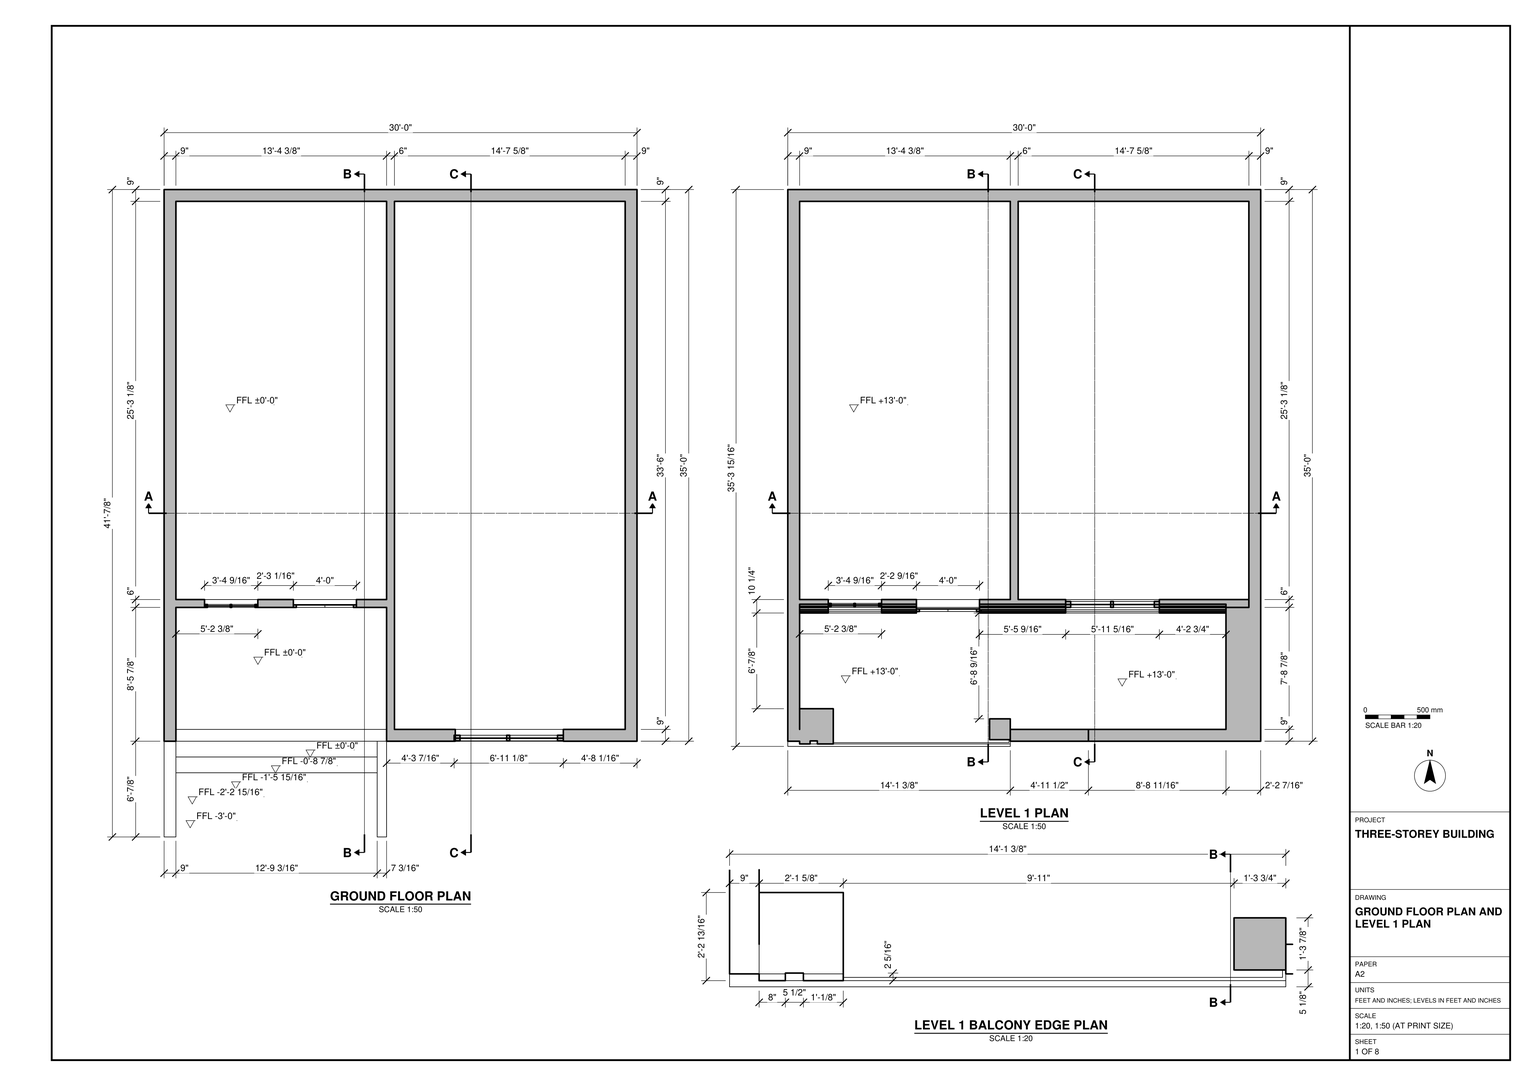
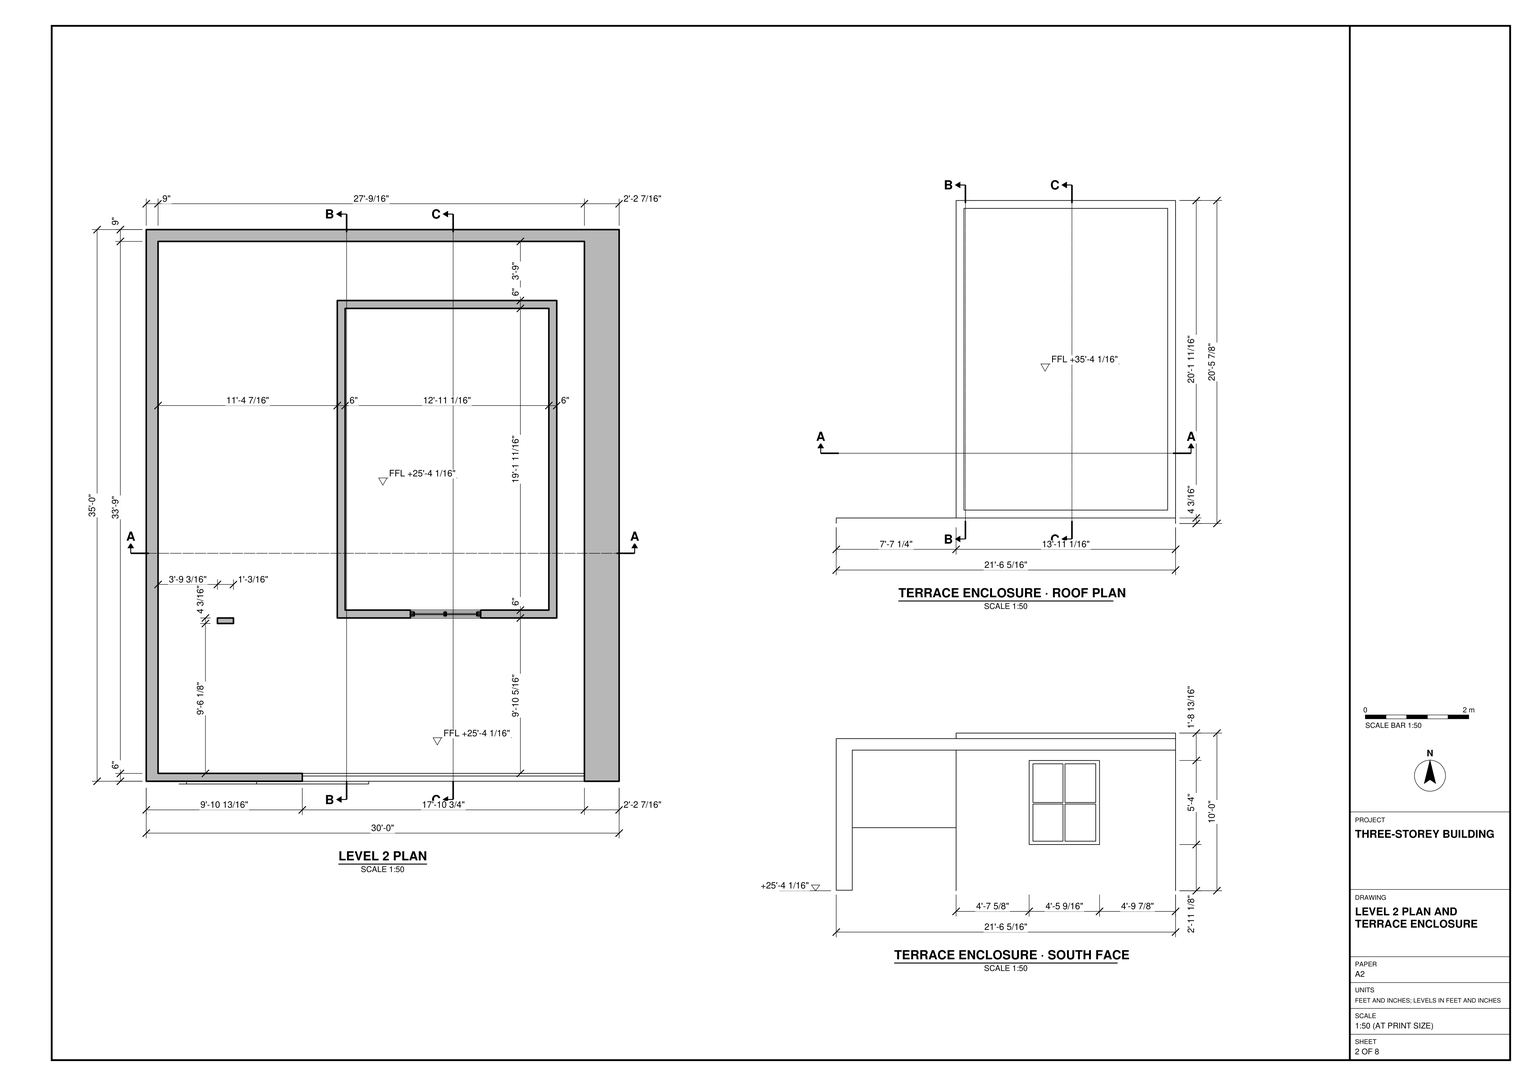
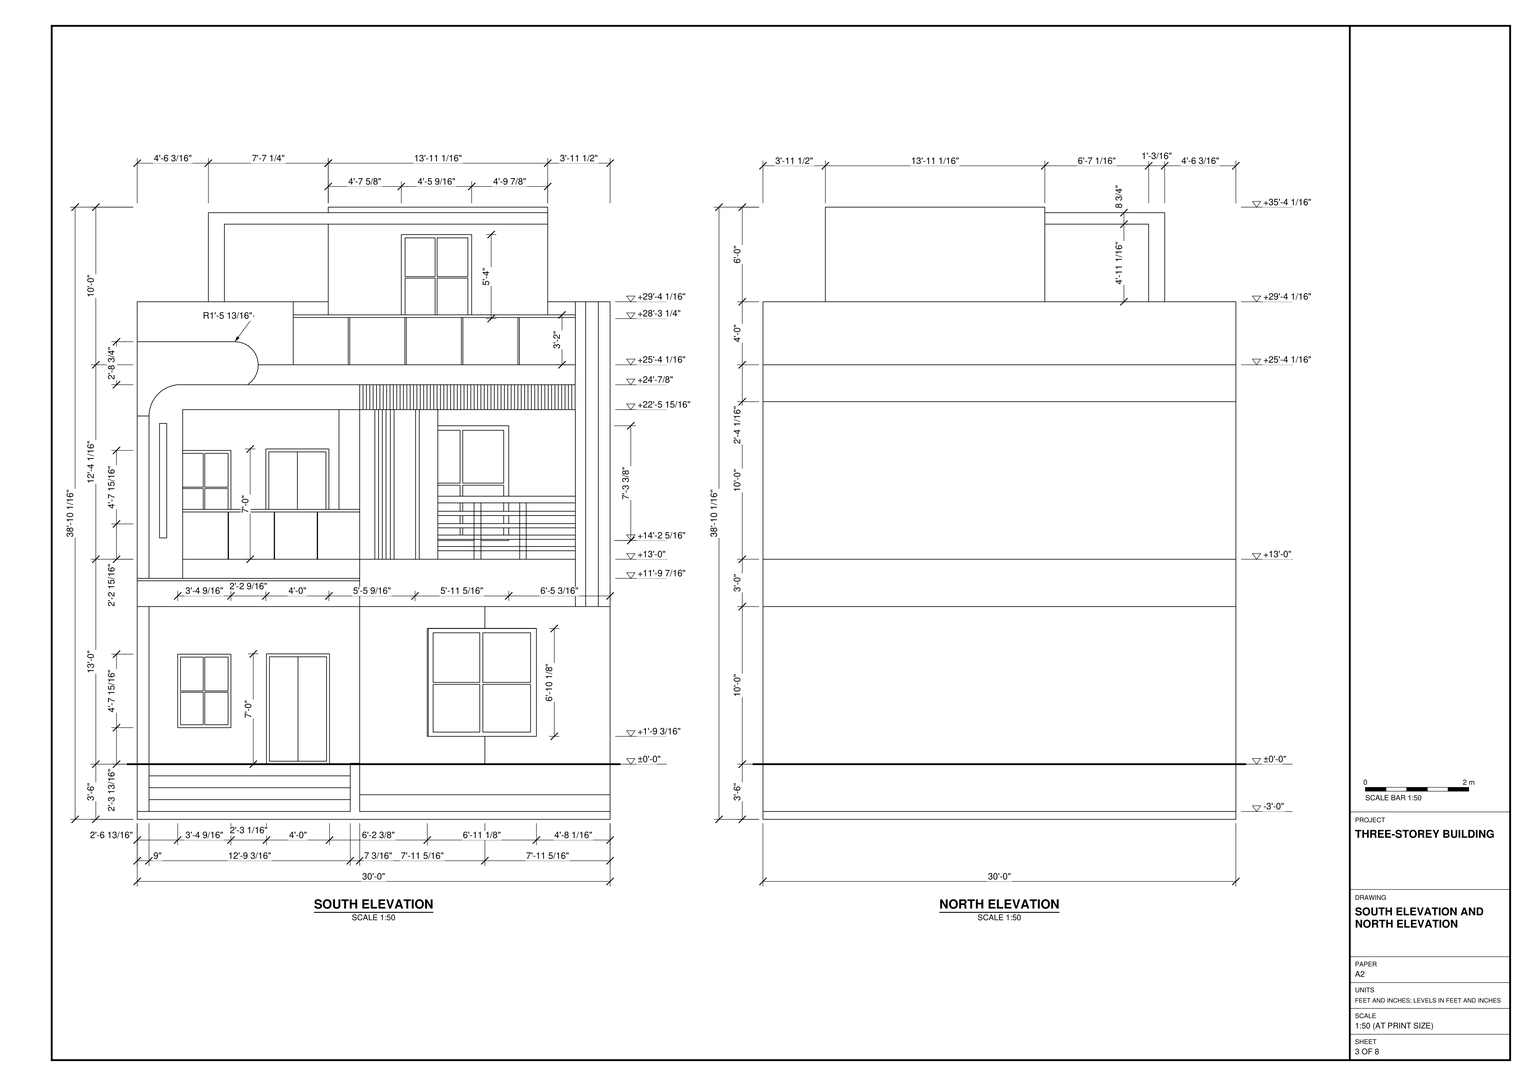
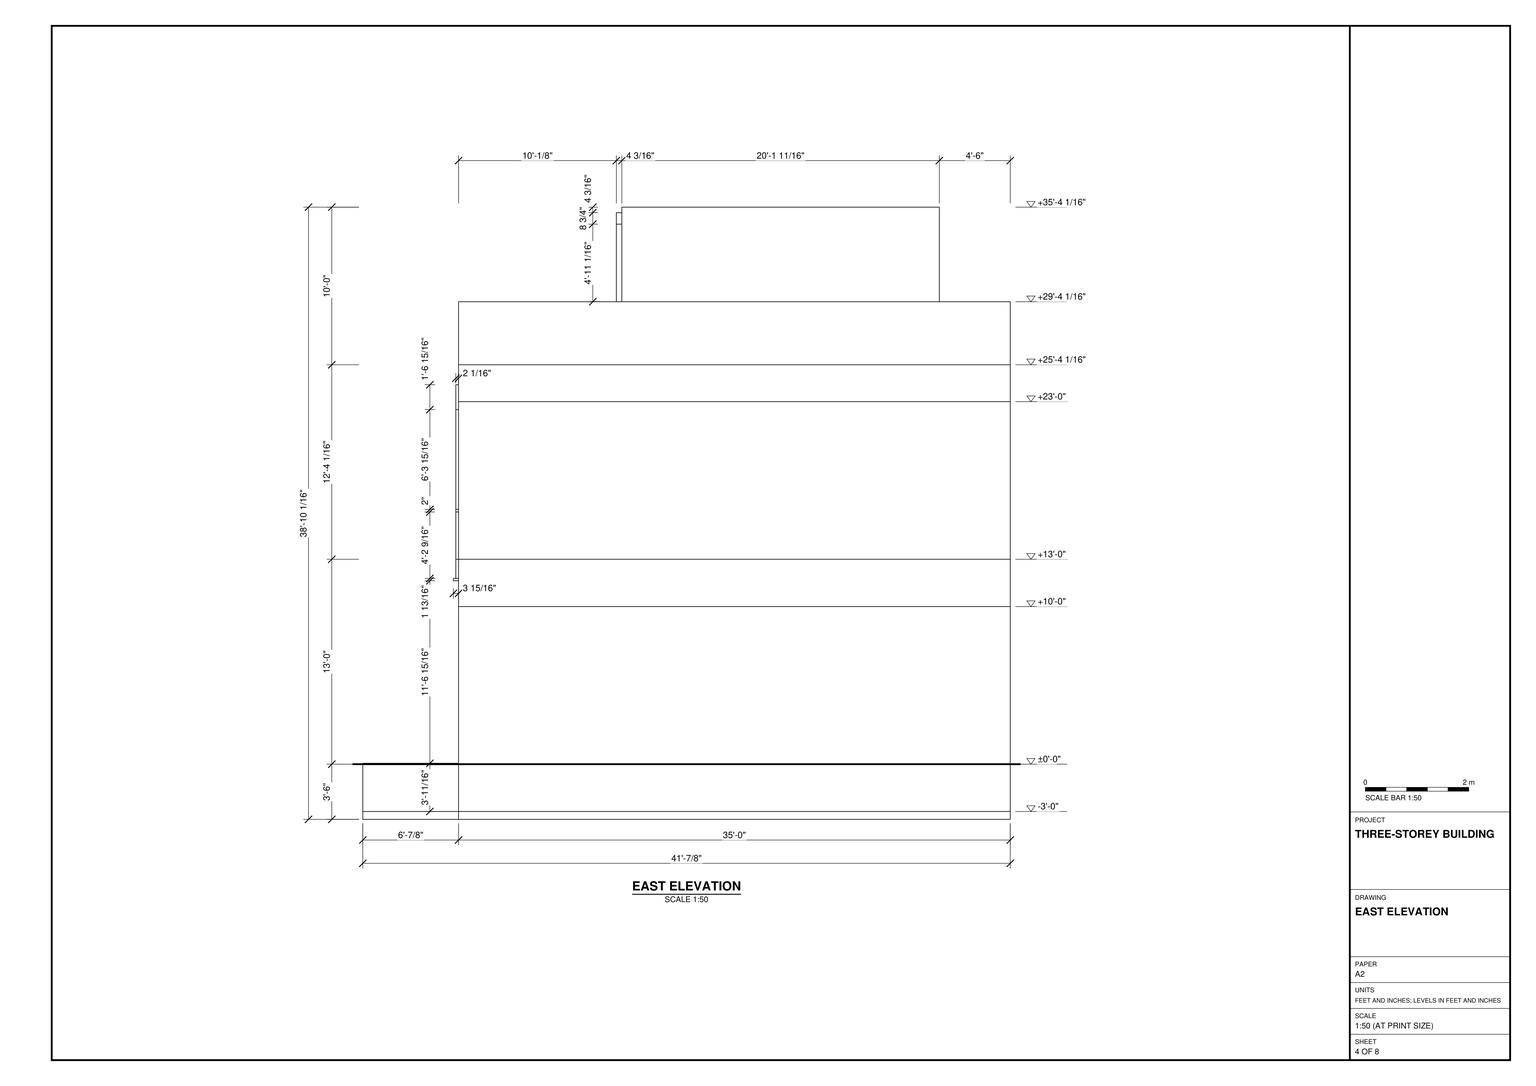
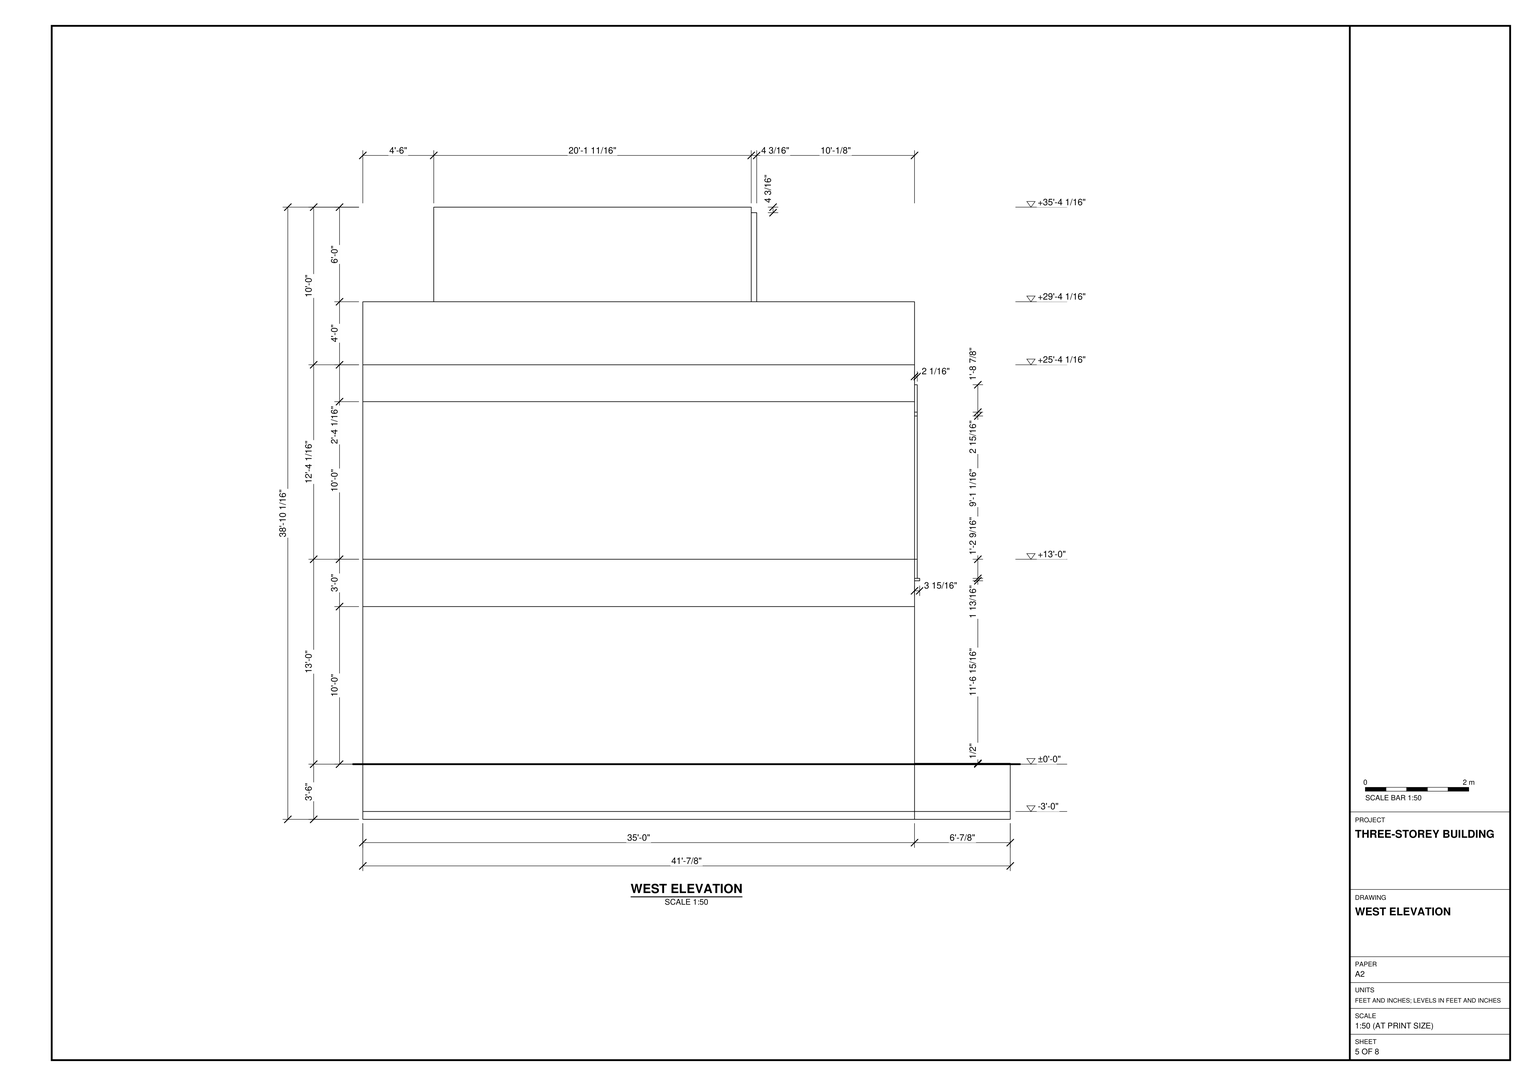
Build the three-storey building in SketchUp from task_files/diagram_01.pdf. Work in feet and inches. The overall model is 30'-0" wide, 41'-7/8" deep including the entrance steps, and 38'-10 1/16" high. Set the ground floor at ±0'-0", Level 1 at +13'-0", and the Level 2 terrace at +25'-4 1/16".

Lay out the two lower floors with the 9" perimeter walls and 6" internal walls shown in plan. On the south side, model the steps and landing leading to the recessed entrance in the left bay. Place the smaller window beside the entrance and the larger window in the projecting right bay. Above, set the doors and windows back behind the balcony. Follow the south elevation for the balcony guards, the curved return of the outer frame, and the strip of closely spaced vertical ribs. Keep the north elevation blank apart from the horizontal divisions shown.

Model the floor slabs, terrace parapets and railing, and the set-back terrace enclosure with its flat roof, south-facing window and open frame extension. Keep the walls, slabs and roof in separate groups or components. Treat each furniture or joinery piece shown as a separate group or component, and use components for repeated parts. Decor and loose items may be any suitable library components. Save one SketchUp model as output_files/three_storey_building_with_a_balcony_and_roof_terrace.skp.

# SketchUp Ruby script. Lengths in inches.
U = 1.inch
M = Sketchup.active_model
def pt(a) = Geom::Point3d.new(a.map { |v| v * U })
def face(e, loops, mat)
  f = e.add_face(loops[0].map { |a| pt(a) })
  loops[1..].each { |l| e.add_face(l.map { |a| pt(a) }).erase! }
  f.material = f.back_material = mat if mat
  f
end
# faces: each face lists its corners as indices into pts; further lists are holes
def faces(e, pts, list, mat = nil) = list.each { |f| face(e, (f[0].is_a?(Array) ? f : [f]).map { |l| l.map { |i| pts[i] } }, mat) }
# xy, xz, yz: faces in a plane at the given z, y or x. An outline is a flat list of corners, or four numbers for a rectangle; further outlines are holes
def ring(l) = l.size == 4 ? [[l[0], l[1]], [l[2], l[1]], [l[2], l[3]], [l[0], l[3]]] : l.each_slice(2).to_a
def flat(e, list, mat, &to3) = list.each { |f| face(e, (f[0].is_a?(Array) ? f : [f]).map { |l| ring(l).map { |u, v| to3.(u, v) } }, mat) }
def xy(e, z, list, mat = nil) = flat(e, list, mat) { |x, y| [x, y, z] }
def xz(e, y, list, mat = nil) = flat(e, list, mat) { |x, z| [x, y, z] }
def yz(e, x, list, mat = nil) = flat(e, list, mat) { |y, z| [x, y, z] }
def lines(e, pts, list) = list.each { |a, b| e.add_line(pt(pts[a]), pt(pts[b])) }
# prism: a flat outline (further loops are holes) pulled along v
def prism(e, loops, v, mat = nil)
  f = face(e, loops, mat); d = Geom::Vector3d.new(v.map { |x| x * U })
  f.pushpull(f.normal.samedirection?(d) ? d.length : -d.length)
end
def box(e, o, s, mat = nil) = prism(e, [[o, [o[0] + s[0], o[1], o[2]], [o[0] + s[0], o[1] + s[1], o[2]], [o[0], o[1] + s[1], o[2]]]], [0, 0, s[2]], mat)
def at(x, y, z, deg = 0) = Geom::Transformation.translation(pt([x, y, z])) * Geom::Transformation.rotation(ORIGIN, Z_AXIS, deg.degrees)
def axes(o, x, y, z) = Geom::Transformation.new([*x, 0, *y, 0, *z, 0, *pt(o).to_a, 1])
def part(name) = M.definitions.add(name)
# library, detail: a bought-in or finely detailed component or shape, given as its bounding box
def library(name, o, s) = part(name).tap { |d| box(d.entities, o, s) }
def detail(e, o, s) = box(e.add_group.entities, o, s)
def put(e, d, t, mat = nil) = e.add_instance(d, t).tap { |i| i.material = mat if mat }
def group(e, t, mat = nil) = e.add_group.tap { |g| g.transformation = t; g.material = mat if mat }.entities
root = M.entities
M.materials.add("[0111_SlateGray]").color = [112, 128, 144]
M.materials.add("[Color B08]").color = [102, 25, 0]
M.materials.add("[Color C08]").color = [102, 72, 0]
M.materials.add("[Color D07]").color = [153, 114, 85]
M.materials.add("[Color E01]").color = [255, 255, 204]
M.materials.add("[Color E07]1").color = [153, 153, 106]
M.materials.add("[Color M02]").color = [198, 198, 198]
M.materials.add("[Color M03]").color = [170, 170, 170]
M.materials.add("[Color M04]").color = [142, 142, 142]
M.materials.add("[Color M05]").color = [114, 114, 114]
M.materials.add("[Color M06]").color = [86, 86, 86]
M.materials.add("[Color M07]").color = [58, 58, 58]
M.materials.add("[Color M08]").color = [30, 30, 30]
M.materials.add("[Pavers with Grass Brick]").color = [187, 192, 176]
M.materials.add("[Translucent Glass Gray]").color = [128, 128, 128]
M.materials["[Translucent Glass Gray]"].alpha = 0.5
c1 = part("Group\#1")
xy(c1.entities,0,[[0,0,61.8125,2.1875],[0,2.1875,61.8125,4.5625]],"[Color B08]")
xy(c1.entities,3.32,[[3.32,0,29.72,2.1875],[31.47,0,58.49,2.1875],[3.32,2.1875,29.72,4.5625],[31.47,2.1875,58.49,4.5625]],"[Color B08]")
xy(c1.entities,40.35,[[3.32,0,29.72,2.1875],[31.47,0,58.49,2.1875],[3.32,2.1875,29.72,4.5625],[31.47,2.1875,58.49,4.5625]],"[Color B08]")
xy(c1.entities,41.875,[[3.32,0,29.72,2.1875],[31.47,0,58.49,2.1875],[3.32,2.1875,29.72,4.5625],[31.47,2.1875,58.49,4.5625]],"[Color B08]")
xy(c1.entities,80.43,[[3.32,0,29.72,2.1875],[31.47,0,58.49,2.1875],[3.32,2.1875,29.72,4.5625],[31.47,2.1875,58.49,4.5625]],"[Color B08]")
xy(c1.entities,83.75,[[0,0,61.8125,2.1875],[0,2.1875,61.8125,4.5625]],"[Color B08]")
xz(c1.entities,0,[[[0,0,61.8125,83.75],[31.47,41.875,58.49,80.43],[3.32,41.875,29.72,80.43],[31.47,3.32,58.49,40.35],[3.32,3.32,29.72,40.35]]],"[Color B08]")
xz(c1.entities,2.1875,[[[0,0,61.8125,83.75],[31.47,41.875,58.49,80.43],[3.32,41.875,29.72,80.43],[31.47,3.32,58.49,40.35],[3.32,3.32,29.72,40.35]]],"[Color B08]")
xz(c1.entities,2.1875,[[3.32,3.32,29.72,40.35],[31.47,3.32,58.49,40.35],[3.32,41.875,29.72,80.43],[31.47,41.875,58.49,80.43]],"[Translucent Glass Gray]")
xz(c1.entities,4.5625,[[[0,0,61.8125,83.75],[31.47,41.875,58.49,80.43],[3.32,41.875,29.72,80.43],[31.47,3.32,58.49,40.35],[3.32,3.32,29.72,40.35]]],"[Color B08]")
yz(c1.entities,0,[[0,0,2.1875,83.75],[2.1875,0,4.5625,83.75]],"[Color B08]")
yz(c1.entities,3.32,[[0,3.32,2.1875,40.35],[2.1875,3.32,4.5625,40.35],[0,41.875,2.1875,80.43],[2.1875,41.875,4.5625,80.43]],"[Color B08]")
yz(c1.entities,29.72,[[0,3.32,2.1875,40.35],[2.1875,3.32,4.5625,40.35],[0,41.875,2.1875,80.43],[2.1875,41.875,4.5625,80.43]],"[Color B08]")
yz(c1.entities,31.47,[[0,3.32,2.1875,40.35],[2.1875,3.32,4.5625,40.35],[0,41.875,2.1875,80.43],[2.1875,41.875,4.5625,80.43]],"[Color B08]")
yz(c1.entities,58.49,[[0,3.32,2.1875,40.35],[2.1875,3.32,4.5625,40.35],[0,41.875,2.1875,80.43],[2.1875,41.875,4.5625,80.43]],"[Color B08]")
yz(c1.entities,61.8125,[[0,0,2.1875,83.75],[2.1875,0,4.5625,83.75]],"[Color B08]")
c2 = part("Group\#2")
xy(c2.entities,0,[[0,0,48,1.9375]],"[Color B08]")
xy(c2.entities,2.25,[[2.25,0,24,1.9375],[24,0,45.75,1.9375]],"[Color B08]")
xy(c2.entities,81.75,[[2.25,0,24,1.9375],[24,0,45.75,1.9375]],"[Color B08]")
xy(c2.entities,84,[[0,0,48,1.9375]],"[Color B08]")
xz(c2.entities,0,[[[0,0,48,84],[2.25,2.25,45.75,81.75]]],"[Color B08]")
xz(c2.entities,1.9375,[[[0,0,48,84],[2.25,2.25,45.75,81.75]]],"[Color B08]")
xz(c2.entities,1.9375,[[2.25,2.25,24,81.75],[24,2.25,45.75,81.75]],"[Color D07]")
yz(c2.entities,0,[[0,0,1.9375,84]],"[Color B08]")
yz(c2.entities,2.25,[[0,2.25,1.9375,81.75]],"[Color B08]")
yz(c2.entities,45.75,[[0,2.25,1.9375,81.75]],"[Color B08]")
yz(c2.entities,48,[[0,0,1.9375,84]],"[Color B08]")
xy(root,0,[[0,0,360,72.875],[0,72.875,360,492.875]])
xy(root,6,[[0,0,9,72.875],[9,0,162.21,24.875],[9,24.875,162.21,36.875],[9,36.875,162.21,72.875],[0,72.875,360,492.875]])
xy(root,6,[[169.375,0,360,72.875]],"[Pavers with Grass Brick]")
xy(root,15.04,[[9,24.875,162.21,36.875]])
xy(root,24.08,[[9,36.875,162.21,48.875]])
xy(root,33.12,[[9,48.875,162.21,60.875]])
xy(root,42,[[9,60.875,162.21,72.875],[9,72.875,169.375,81.875],[9,81.875,169.375,81.875,169.375,174.75,146.42,174.75,146.42,180.75,98.42,180.75,98.42,174.75,9,174.75],[175.375,81.875,351,483.875],[9,180.75,169.375,483.875]])
xy(root,42.16,[[0,0,9,72.875]])
xy(root,42.6875,[[162.21,0,169.375,72.875]])
xy(root,63.17,[[221.67,72.875,303.92,81.875]])
xy(root,69.81,[[30.8,174.75,71.37,180.75]])
xy(root,125.74,[[30.8,174.75,71.37,180.75]])
xy(root,126,[[98.42,174.75,146.42,180.75]])
xy(root,145.42,[[221.67,72.875,303.92,81.875]])
xy(root,156,[[175.375,81.875,351,483.875],[9,180.75,169.375,483.875]])
xy(root,162,[[[0,72.875,0,492.875,360,492.875,360,72.875,169.375,72.875,169.375,174.75,9,174.75,9,72.875],[175.375,81.875,351,483.875],[9,180.75,169.375,483.875]],[9,72.875,169.375,174.75],[175.375,81.875,351,483.875],[9,180.75,169.375,483.875]])
xy(root,181.62,[[0,68.9375,9,72.875],[9,68.9375,34.625,72.875],[34.625,68.9375,169.375,72.875]])
xy(root,183.45,[[0,68.9375,169.375,68.9375,169.375,70.8125,9,70.8125,9,72.875,0,72.875],[9,70.8125,34.625,72.875],[34.625,70.8125,169.375,72.875]])
xy(root,198,[[34.625,70.8125,69.17,71.8125],[69.17,70.8125,69.55,71.8125],[69.55,70.8125,104.23,71.8125],[104.23,70.8125,104.61,71.8125],[104.61,70.8125,136.99,71.8125],
  [136.99,70.8125,137.375,71.8125],[137.375,70.8125,137.375,71.8125,168.375,71.8125,168.375,74.0625,169.375,74.0625,169.375,70.8125],[34.625,71.8125,168.375,71.8125,168.375,74.0625,153.61,74.0625,153.61,89.9375,169.375,89.9375,169.375,81.875,333.5625,81.875,333.5625,170.5,145.93,170.5,145.93,174.75,97.93,174.75,97.93,170.5,9,170.5,9,97.65,34.625,97.65],[169.375,72.875,228.85,81.875],[228.85,72.875,254.8,72.875,254.8,75.625,256.43,75.625,256.43,80.375,254.8,80.375,254.8,81.875,228.85,81.875],
  [261.69,72.875,289.24,72.875,289.24,75.625,291.18,75.625,291.18,80.375,289.24,80.375,289.24,81.875,261.69,81.875],[296.13,72.875,333.5625,81.875],[333.5625,81.875,351,174.75],[9,170.5,97.93,171.625],[145.93,170.5,169.375,171.625],
  [169.375,170.5,175.375,171.625],[175.375,170.5,333.5625,171.625],[9,171.625,97.93,172.9375],[145.93,171.625,169.375,172.9375],[169.375,171.625,175.375,172.9375],
  [175.375,171.625,333.5625,172.9375],[9,172.9375,97.93,174.75],[145.93,172.9375,169.375,174.75],[169.375,172.9375,175.375,174.75],[175.375,172.9375,333.5625,174.75],
  [9,174.75,97.93,175.5625],[97.93,174.75,145.93,180.75],[145.93,174.75,169.375,175.5625],[169.375,174.75,175.375,175.5625],[175.375,174.75,333.5625,175.5625],
  [9,175.5625,97.93,177.1875],[145.93,175.5625,169.375,177.1875],[169.375,175.5625,175.375,177.1875],[175.375,175.5625,333.5625,177.1875],[9,180.75,169.375,483.875],
  [175.375,180.75,351,483.875]])
xy(root,198,[[254.8,72.875,261.69,75.625],[289.24,72.875,296.13,75.625],[256.43,75.625,261.69,80.375],[291.18,75.625,296.13,80.375],[254.8,80.375,261.69,81.875],
  [289.24,80.375,296.13,81.875]],"[Color M08]")
xy(root,204.48,[[228.85,75.27,333.66,79.59]],"[Color M07]")
xy(root,207.73,[[228.85,75.27,333.66,79.59]],"[Color M07]")
xy(root,212.28,[[211.52,170.5,282.83,171.625],[211.52,171.625,282.83,172.9375],[211.52,172.9375,282.83,174.75],[211.52,174.75,282.83,175.5625],[211.52,175.5625,282.83,177.1875],
  [211.52,177.1875,282.83,180.75]])
xy(root,213.17,[[228.85,75.27,333.72,79.59]],"[Color M07]")
xy(root,214.23,[[16.98,70.8125,22.48,73.125]])
xy(root,216.42,[[228.85,75.27,333.72,79.59]],"[Color M07]")
xy(root,221.92,[[228.85,75.27,334.79,79.59]],"[Color M07]")
xy(root,224.93,[[30.8,170.5,71.37,171.625],[30.8,171.625,71.37,172.9375],[30.8,172.9375,71.37,174.75],[30.8,174.75,71.37,175.5625],[30.8,175.5625,71.37,177.1875],
  [30.8,177.1875,71.37,180.75]])
xy(root,225.17,[[228.85,75.27,334.79,79.59]],"[Color M07]")
xy(root,231.3,[[228.85,75.27,333.5625,79.59]],"[Color M07]")
xy(root,234,[[34.625,70.8125,69.17,71.8125],[69.17,70.8125,69.55,71.8125],[69.55,70.8125,104.23,71.8125],[104.23,70.8125,104.61,71.8125],[104.61,70.8125,136.99,71.8125],
  [136.99,70.8125,137.375,71.8125],[137.375,70.8125,137.375,71.8125,168.375,71.8125,168.375,74.0625,169.375,74.0625,169.375,70.8125]],"[Color M04]")
xy(root,234.55,[[228.85,75.27,333.5625,79.59]],"[Color M07]")
xy(root,236,[[34.625,70.8125,169.375,70.8125,169.375,74.0625,168.375,74.0625,168.375,71.8125,34.625,71.8125]],"[Color M04]")
xy(root,240.93,[[228.85,72.875,228.85,81.875,254.8,81.875,254.8,80.375,256.43,80.375,256.43,75.625,254.8,75.625,254.8,72.875],[254.8,72.875,261.69,75.625],[261.69,72.875,261.69,81.875,289.24,81.875,289.24,80.375,291.18,80.375,291.18,75.625,289.24,75.625,289.24,72.875],[289.24,72.875,296.13,75.625],[296.13,72.875,333.5625,81.875],
  [256.43,75.625,261.69,80.375],[291.18,75.625,296.13,80.375],[254.8,80.375,261.69,81.875],[289.24,80.375,296.13,81.875]],"[Color M08]")
xy(root,246,[[228.85,72.875,333.5625,81.875]],"[Color M07]")
xy(root,280.87,[[30.8,170.5,71.37,171.625],[30.8,171.625,71.37,172.9375],[30.8,172.9375,71.37,174.75],[30.8,174.75,71.37,175.5625],[30.8,175.5625,71.37,177.1875],
  [30.8,177.1875,71.37,180.75]])
xy(root,282,[[97.93,170.5,145.93,171.625],[97.93,171.625,145.93,172.9375],[97.93,172.9375,145.93,174.75],[97.93,174.75,145.93,175.5625],[97.93,175.5625,145.93,177.1875],
  [97.93,177.1875,145.93,180.75]])
xy(root,299.66,[[211.52,170.5,282.83,171.625],[211.52,171.625,282.83,172.9375],[211.52,172.9375,282.83,174.75],[211.52,174.75,282.83,175.5625],[211.52,175.5625,282.83,177.1875],
  [211.52,177.1875,282.83,180.75]])
xy(root,301.42,[[16.98,70.8125,22.48,73.125]])
xy(root,311.9375,[[34.625,70.8125,34.625,97.65,9,97.65,9,170.5,169.375,170.5,169.375,89.9375,153.61,89.9375,153.61,70.8125],[153.61,70.8125,169.375,74.0625],[169.375,72.875,228.85,81.875],[228.85,72.875,228.85,81.875,169.375,81.875,169.375,170.5,333.5625,170.5,333.5625,72.875],[153.61,74.0625,169.375,89.9375],
  [9,170.5,169.375,171.625],[169.375,170.5,333.5625,171.625],[9,171.625,169.375,172.9375],[169.375,171.625,333.5625,172.9375],[9,172.9375,169.375,174.75],
  [169.375,172.9375,333.5625,174.75],[9,174.75,169.375,175.5625],[169.375,174.75,333.5625,175.5625],[9,175.5625,169.375,177.1875],[169.375,175.5625,333.5625,177.1875]])
xy(root,312,[[9,180.75,169.375,483.875],[175.375,180.75,351,483.875]])
xy(root,318,[[9,180.75,351,483.875]])
xy(root,330.875,[[30.64,70.8125,83.99,72.875],[83.99,70.8125,169.375,72.875]])
xy(root,337.07,[[9,180.75,351,483.875]])
xy(root,346.07,[[118.8,72.875,333.5625,76.875],[118.8,76.875,160.66,78.875],[160.66,76.875,161.79,78.875],[161.79,76.875,203.73,78.875],[203.73,76.875,204.85,78.875],
  [204.85,76.875,246.79,78.875],[246.79,76.875,247.92,78.875],[247.92,76.875,289.85,78.875],[289.85,76.875,290.98,78.875],[290.98,76.875,333.5625,78.875],
  [[9,78.875,333.5625,483.875],[145.4375,197.1875,312.5,438.875]],[333.5625,78.875,351,174.75],[333.5625,174.75,351,180.75],[333.5625,180.75,351,483.875],[[145.4375,197.1875,312.5,438.875],[151.4375,203.1875,306.5,432.875]],
  [151.4375,203.1875,306.5,432.875]])
xy(root,346.43,[[54.1875,193,66.4,197.1875]],"[Color M06]")
xy(root,381.23,[[201.06,197.1875,254.62,203.1875]])
xy(root,382.07,[[160.66,76.875,161.79,78.875],[203.73,76.875,204.85,78.875],[246.79,76.875,247.92,78.875],[289.85,76.875,290.98,78.875]],"[Color C08]")
xy(root,382.07,[[118.8,76.875,160.66,78.875],[161.79,76.875,203.73,78.875],[204.85,76.875,246.79,78.875],[247.92,76.875,289.85,78.875],[290.98,76.875,333.5625,78.875]],"[Color M06]")
xy(root,384.07,[[118.8,76.875,333.5625,78.875]],"[Color M06]")
xy(root,394.07,[[0,72.875,118.8,72.875,118.8,78.875,9,78.875,9,483.875,333.5625,483.875,333.5625,72.875,360,72.875,360,492.875,0,492.875]],"[Color E01]")
xy(root,445.23,[[201.06,197.1875,254.62,203.1875]])
xy(root,453.12,[[66.4,193,312.5,197.1875]],"[Color M06]")
xy(root,460.07,[[151.4375,203.1875,306.5,432.875]])
xy(root,461.87,[[54.1875,193,312.5,197.1875]],"[Color M06]")
xy(root,466.07,[[[145.4375,197.1875,312.5,438.875],[151.4375,203.1875,306.5,432.875]],[151.4375,203.1875,306.5,432.875]])
xz(root,0,[[0,0,360,0,360,6,169.375,6,169.375,42.6875,162.21,42.6875,162.21,6,0,6],[0,6,9,42.16]])
xz(root,24.875,[[9,6,162.21,15.04]])
xz(root,36.875,[[9,15.04,162.21,24.08]])
xz(root,48.875,[[9,24.08,162.21,33.12]])
xz(root,60.875,[[9,33.12,162.21,42]])
xz(root,68.9375,[[0,181.62,169.375,183.45]])
xz(root,70.8125,[[34.625,183.45,169.375,198],[69.17,198,69.55,234],[104.23,198,104.61,234],[136.99,198,137.375,234]],"[Color C08]")
xz(root,70.8125,[[[9,183.45,34.625,183.45,34.625,311.9375,169.375,311.9375,169.375,330.875,30.64,330.875,27.74,330.42,24.91,329.61,22.21,328.46,19.67,326.98,17.33,325.21,15.22,323.16,13.38,320.87,11.84,318.37,10.61,315.7,9.72,312.9,9.18,310.01,9,307.08],[16.98,214.23,22.48,301.42]]],"[Color M03]")
xz(root,70.8125,[[34.625,234,169.375,236]],"[Color M04]")
xz(root,70.8125,[[34.625,198,69.17,234],[69.55,198,104.23,234],[104.61,198,136.99,234],[137.375,198,169.375,234]],"[Translucent Glass Gray]")
xz(root,71.8125,[[168.0625,198,168.375,234]])
xz(root,71.8125,[[69.17,198,69.55,234],[104.23,198,104.61,234],[136.99,198,137.375,234]],"[Color C08]")
xz(root,71.8125,[[34.625,234,168.0625,236],[168.0625,234,168.375,236]],"[Color M04]")
xz(root,71.8125,[[34.625,198,69.17,234],[69.55,198,104.23,234],[104.61,198,136.99,234],[137.375,198,168.0625,234]],"[Translucent Glass Gray]")
xz(root,72.875,[[0,0,360,6],[0,6,9,42.16],[9,6,162.21,33.12],[162.21,6,169.375,42],[169.375,18.77,360,42],
  [9,33.12,162.21,42],[162.21,42,169.375,42.6875],[0,162,169.375,181.62],[333.5625,162,341.39,162,341.39,394.07,333.5625,394.07,333.5625,346.07,333.375,330.875,333.375,311.9375,333.5625,311.9375],[351.02,162,360,394.07],
  [0,181.62,169.375,183.45],[169.375,198,180.91,311.9375],[183.74,198,186.59,311.9375],[189.42,198,192.72,311.9375],[195.55,198,211.91,311.9375],
  [214.74,198,228.85,311.9375],[169.375,311.9375,171.9375,330.875],[171.9375,311.9375,174.5,330.875],[174.5,311.9375,177.0625,330.875],[177.0625,311.9375,179.625,330.875],
  [179.625,311.9375,182.1875,330.875],[182.1875,311.9375,184.75,330.875],[184.75,311.9375,187.3125,330.875],[187.3125,311.9375,189.875,330.875],[189.875,311.9375,192.4375,330.875],
  [192.4375,311.9375,195,330.875],[195,311.9375,197.5625,330.875],[197.5625,311.9375,200.125,330.875],[200.125,311.9375,202.6875,330.875],[202.6875,311.9375,205.25,330.875],
  [205.25,311.9375,207.8125,330.875],[207.8125,311.9375,210.375,330.875],[210.375,311.9375,212.9375,330.875],[212.9375,311.9375,215.5,330.875],[215.5,311.9375,218.0625,330.875],
  [218.0625,311.9375,220.625,330.875],[220.625,311.9375,223.1875,330.875],[223.1875,311.9375,225.75,330.875],[225.75,311.9375,228.3125,330.875],[228.3125,311.9375,230.875,330.875],
  [230.875,311.9375,233.4375,330.875],[233.4375,311.9375,236,330.875],[236,311.9375,238.5625,330.875],[238.5625,311.9375,241.125,330.875],[241.125,311.9375,243.6875,330.875],
  [243.6875,311.9375,246.25,330.875],[246.25,311.9375,248.8125,330.875],[248.8125,311.9375,251.375,330.875],[251.375,311.9375,253.9375,330.875],[253.9375,311.9375,256.5,330.875],
  [256.5,311.9375,259.0625,330.875],[259.0625,311.9375,261.625,330.875],[261.625,311.9375,264.1875,330.875],[264.1875,311.9375,266.75,330.875],[266.75,311.9375,269.3125,330.875],
  [269.3125,311.9375,271.875,330.875],[271.875,311.9375,274.4375,330.875],[274.4375,311.9375,277,330.875],[277,311.9375,279.5625,330.875],[279.5625,311.9375,282.125,330.875],
  [282.125,311.9375,284.6875,330.875],[284.6875,311.9375,287.25,330.875],[287.25,311.9375,289.8125,330.875],[289.8125,311.9375,292.375,330.875],[292.375,311.9375,294.9375,330.875],
  [294.9375,311.9375,297.5,330.875],[297.5,311.9375,300.0625,330.875],[300.0625,311.9375,302.625,330.875],[302.625,311.9375,305.1875,330.875],[305.1875,311.9375,307.75,330.875],
  [307.75,311.9375,310.3125,330.875],[310.3125,311.9375,312.875,330.875],[312.875,311.9375,315.4375,330.875],[315.4375,311.9375,318,330.875],[318,311.9375,320.5625,330.875],
  [320.5625,311.9375,323.125,330.875],[323.125,311.9375,325.6875,330.875],[325.6875,311.9375,328.25,330.875],[328.25,311.9375,330.8125,330.875],[330.8125,311.9375,333.375,330.875]])
xz(root,72.875,[[169.375,162,333.5625,198],[0,307.08,9,307.08,9.18,310.01,9.72,312.9,10.61,315.7,11.84,318.37,13.38,320.87,15.22,323.16,17.33,325.21,19.67,326.98,22.21,328.46,24.91,329.61,27.74,330.42,30.64,330.875,83.99,330.875,86.96,333.26,89.34,336.22,91.05,339.625,91.99,343.3125,92.09,346.07,92.125,347.11,91.45,350.86,89.99,354.375,87.82,357.5,85.04,360.09,81.77,362.03,78.16,363.24,74.375,363.64,0,363.64]],"[0111_SlateGray]")
xz(root,72.875,[[83.99,330.875,333.375,330.875,333.5625,346.07,92.09,346.07,91.99,343.3125,91.05,339.625,89.34,336.22,86.96,333.26]],"[Color C08]")
xz(root,72.875,[[0,42.16,9,162],[0,183.45,9,307.08],[92.09,346.07,118.8,346.07,118.8,394.07,0,394.07,0,363.64,74.375,363.64,78.16,363.24,81.77,362.03,85.04,360.09,87.82,357.5,89.99,354.375,91.45,350.86,92.125,347.11]],"[Color E01]")
xz(root,72.875,[[264.6875,42,360,42,360,162,264.6875,162,264.6875,145.42,303.92,145.42,303.92,63.17,264.6875,63.17]],"[Color E07]1")
xz(root,72.875,[[169.375,42,264.6875,42,264.6875,63.17,221.67,63.17,221.67,145.42,264.6875,145.42,264.6875,162,169.375,162]],"[Color M02]")
xz(root,72.875,[[169.375,6,360,18.77],[341.39,162,351.02,394.07]],"[Color M03]")
xz(root,72.875,[[180.91,198,183.74,311.9375],[186.59,198,189.42,311.9375],[192.72,198,195.55,311.9375],[211.91,198,214.74,311.9375]],"[Color M04]")
xz(root,72.875,[[228.85,240.93,333.5625,246]],"[Color M07]")
xz(root,73.125,[[16.98,214.23,22.48,301.42]])
xz(root,74.0625,[[168.375,198,169.375,234]])
xz(root,74.0625,[[153.61,198,168.375,198,168.375,236,169.375,236,169.375,311.9375,153.61,311.9375]],"[Color M03]")
xz(root,74.0625,[[168.375,234,169.375,236]],"[Color M04]")
xz(root,75.27,[[228.85,204.48,333.66,207.73],[228.85,213.17,333.72,216.42],[228.85,221.92,334.79,225.17],[228.85,231.3,333.5625,234.55]],"[Color M07]")
xz(root,75.625,[[256.43,198,261.69,240.93],[291.18,198,296.13,240.93]],"[Color M07]")
xz(root,76.875,[[160.66,346.07,161.79,382.07],[203.73,346.07,204.85,382.07],[246.79,346.07,247.92,382.07],[289.85,346.07,290.98,382.07]],"[Color C08]")
xz(root,76.875,[[118.8,382.07,333.5625,384.07]],"[Color M06]")
xz(root,76.875,[[118.8,346.07,160.66,382.07],[161.79,346.07,203.73,382.07],[204.85,346.07,246.79,382.07],[247.92,346.07,289.85,382.07],[290.98,346.07,333.5625,382.07]],"[Translucent Glass Gray]")
xz(root,78.875,[[160.66,346.07,161.79,382.07],[203.73,346.07,204.85,382.07],[246.79,346.07,247.92,382.07],[289.85,346.07,290.98,382.07]],"[Color C08]")
xz(root,78.875,[[9,346.07,118.8,394.07]],"[Color E01]")
xz(root,78.875,[[118.8,382.07,121.17,384.07],[121.17,382.07,333.5625,384.07]],"[Color M06]")
xz(root,78.875,[[118.8,346.07,160.66,382.07],[161.79,346.07,203.73,382.07],[204.85,346.07,246.79,382.07],[247.92,346.07,289.85,382.07],[290.98,346.07,333.5625,382.07]],"[Translucent Glass Gray]")
xz(root,79.59,[[228.85,204.48,333.66,207.73],[228.85,213.17,333.72,216.42],[228.85,221.92,334.79,225.17],[228.85,231.3,333.5625,234.55]],"[Color M07]")
xz(root,80.375,[[256.43,198,261.69,240.93],[291.18,198,296.13,240.93]],"[Color M07]")
xz(root,81.875,[[[175.375,42,351,156],[221.67,63.17,303.92,145.42]],[175.375,156,351,162],[175.375,162,351,198],[169.375,198,175.375,311.9375],[175.375,198,228.85,311.9375]])
xz(root,81.875,[[228.85,240.93,333.5625,246]],"[Color M08]")
xz(root,89.9375,[[153.61,198,169.375,311.9375]])
xz(root,97.65,[[9,198,34.625,311.9375],[9,311.9375,34.625,318]])
xz(root,170.5,[[[9,198,97.93,198,97.93,282,145.93,282,145.93,198,333.5625,198,333.5625,311.9375,9,311.9375],[211.52,212.28,282.83,299.66],[30.8,224.93,71.37,280.87]]],"[Color M02]")
xz(root,171.625,[[[9,198,9,311.9375,333.5625,311.9375,333.5625,198,145.93,198,145.93,282,97.93,282,97.93,198],[211.52,212.28,282.83,299.66],[30.8,224.93,71.37,280.87]]])
xz(root,172.9375,[[[9,198,9,311.9375,333.5625,311.9375,333.5625,198,145.93,198,145.93,282,97.93,282,97.93,198],[211.52,212.28,282.83,299.66],[30.8,224.93,71.37,280.87]]])
xz(root,174.75,[[[9,42,98.42,42,98.42,126,146.42,126,146.42,42,169.375,42,169.375,162,9,162],[30.8,69.81,71.37,125.74]],[9,162,169.375,198],[[9,198,97.93,198,97.93,282,145.93,282,145.93,198,333.5625,198,333.5625,311.9375,9,311.9375],[211.52,212.28,282.83,299.66],[30.8,224.93,71.37,280.87]],[333.5625,198,351,311.9375],[9,311.9375,169.375,318]])
xz(root,175.5625,[[[9,198,9,311.9375,333.5625,311.9375,333.5625,198,145.93,198,145.93,282,97.93,282,97.93,198],[211.52,212.28,282.83,299.66],[30.8,224.93,71.37,280.87]]])
xz(root,177.1875,[[[9,198,9,311.9375,333.5625,311.9375,333.5625,198,145.93,198,145.93,282,97.93,282,97.93,198],[211.52,212.28,282.83,299.66],[30.8,224.93,71.37,280.87]]])
xz(root,180.75,[[[9,42,9,156,169.375,156,169.375,42,146.42,42,146.42,126,98.42,126,98.42,42],[30.8,69.81,71.37,125.74]],[9,156,169.375,162],[9,162,169.375,198],[[9,198,9,312,169.375,312,169.375,198,145.93,198,145.93,282,97.93,282,97.93,198],[30.8,224.93,71.37,280.87]],[[175.375,198,351,312],[211.52,212.28,282.83,299.66]],
  [9,312,169.375,318],[175.375,312,351,318],[9,318,351,337.07]])
xz(root,193,[[54.1875,346.43,66.4,346.43,66.4,453.12,312.5,453.12,312.5,461.87,54.1875,461.87]],"[Color M06]")
xz(root,197.1875,[[145.4375,461.87,312.5,466.07]])
xz(root,197.1875,[[[145.4375,346.07,312.5,453.12],[201.06,381.23,254.62,445.23]]],"[Color M02]")
xz(root,197.1875,[[54.1875,346.43,54.1875,461.87,145.4375,461.87,145.4375,453.12,66.4,453.12,66.4,346.43],[145.4375,453.12,312.5,461.87]],"[Color M06]")
xz(root,203.1875,[[[151.4375,346.07,306.5,460.07],[201.06,381.23,254.62,445.23]],[151.4375,460.07,306.5,466.07]])
xz(root,432.875,[[151.4375,346.07,306.5,460.07],[151.4375,460.07,158.1875,466.07],[158.1875,460.07,306.5,466.07]])
xz(root,438.875,[[145.4375,346.07,312.5,466.07]],"[Color M02]")
xz(root,483.875,[[9,42,169.375,156],[175.375,42,351,156],[9,156,28.625,162],[28.625,156,169.375,162],[175.375,156,193.9375,162],
  [193.9375,156,351,162],[9,162,28.625,198],[28.625,162,169.375,198],[175.375,162,193.9375,198],[193.9375,162,351,198],
  [9,198,169.375,312],[175.375,198,351,312],[9,312,44.33,318],[44.33,312,50.33,318],[50.33,312,169.375,318],
  [175.375,312,217.42,318],[217.42,312,226.17,318],[226.17,312,351,318],[9,318,351,337.07],[9,337.07,351,346.07]])
xz(root,483.875,[[9,346.07,333.5625,394.07]],"[Color E01]")
xz(root,492.875,[[0,0,360,6],[0,6,360,42],[0,42,360,162],[0,162,360,198],[0,198,360,318],
  [0,318,360,346.07],[0,346.07,360,394.07]])
yz(root,0,[[0,0,72.875,6],[72.875,0,492.875,6],[0,6,72.875,42.16],[72.875,6,492.875,42],[72.875,42,492.875,162],
  [72.875,162,492.875,198],[68.9375,181.62,72.875,183.45],[72.875,198,492.875,318],[72.875,318,492.875,346.07],[72.875,346.07,492.875,394.07]])
yz(root,9,[[0,6,24.875,6,24.875,15.04,36.875,15.04,36.875,24.08,48.875,24.08,48.875,33.12,60.875,33.12,60.875,42.16,0,42.16],[24.875,6,36.875,15.04],[36.875,6,36.875,24.08,48.875,24.08,48.875,33.12,60.875,33.12,60.875,42,72.875,42,72.875,6],[60.875,42,72.875,42.16],[72.875,42,81.875,162],
  [81.875,42,174.75,162],[180.75,42,483.875,156],[180.75,156,483.875,162],[81.875,162,174.75,198],[180.75,162,483.875,198],
  [70.8125,183.45,72.875,198],[70.8125,198,72.875,307.08],[81.875,198,97.65,318],[97.65,198,170.5,311.9375],[170.5,198,171.625,311.9375],
  [171.625,198,172.9375,311.9375],[172.9375,198,174.75,311.9375],[174.75,198,175.5625,311.9375],[175.5625,198,177.1875,311.9375],[180.75,198,483.875,312],
  [97.65,311.9375,174.75,318],[180.75,312,483.875,318],[81.875,318,174.75,346.07],[180.75,318,483.875,337.07],[180.75,337.07,186.375,346.07],
  [186.375,337.07,483.875,346.07]])
yz(root,9,[[78.875,346.07,483.875,394.07]],"[Color E01]")
yz(root,16.98,[[70.8125,214.23,73.125,301.42]])
yz(root,22.48,[[70.8125,214.23,73.125,301.42]])
yz(root,30.8,[[174.75,69.81,180.75,125.74],[170.5,224.93,171.625,280.87],[171.625,224.93,172.9375,280.87],[172.9375,224.93,174.75,280.87],[174.75,224.93,175.5625,280.87],
  [175.5625,224.93,177.1875,280.87],[177.1875,224.93,180.75,280.87]])
yz(root,34.625,[[70.8125,198,71.8125,234],[71.8125,198,97.65,198,97.65,311.9375,70.8125,311.9375,70.8125,236,71.8125,236]])
yz(root,34.625,[[70.8125,234,71.8125,236]],"[Color M04]")
yz(root,54.1875,[[193,346.43,197.1875,461.87]],"[Color M06]")
yz(root,66.4,[[193,346.43,197.1875,453.12]],"[Color M06]")
yz(root,69.17,[[70.8125,198,71.8125,234]],"[Color C08]")
yz(root,69.55,[[70.8125,198,71.8125,234]],"[Color C08]")
yz(root,71.37,[[174.75,69.81,180.75,125.74],[170.5,224.93,171.625,280.87],[171.625,224.93,172.9375,280.87],[172.9375,224.93,174.75,280.87],[174.75,224.93,175.5625,280.87],
  [175.5625,224.93,177.1875,280.87],[177.1875,224.93,180.75,280.87]])
yz(root,97.93,[[170.5,198,171.625,282],[171.625,198,172.9375,282],[172.9375,198,174.75,282],[174.75,198,175.5625,282],[175.5625,198,177.1875,282],
  [177.1875,198,180.75,282]])
yz(root,98.42,[[174.75,42,180.75,126]])
yz(root,104.23,[[70.8125,198,71.8125,234]],"[Color C08]")
yz(root,104.61,[[70.8125,198,71.8125,234]],"[Color C08]")
yz(root,118.8,[[76.875,346.07,78.875,382.07]])
yz(root,118.8,[[72.875,346.07,76.875,346.07,76.875,384.07,78.875,384.07,78.875,394.07,72.875,394.07]],"[Color E01]")
yz(root,118.8,[[76.875,382.07,78.875,384.07]],"[Color M06]")
yz(root,136.99,[[70.8125,198,71.8125,234]],"[Color C08]")
yz(root,137.375,[[70.8125,198,71.8125,234]],"[Color C08]")
yz(root,145.4375,[[197.1875,346.07,438.875,466.07]],"[Color M02]")
yz(root,145.93,[[170.5,198,171.625,282],[171.625,198,172.9375,282],[172.9375,198,174.75,282],[174.75,198,175.5625,282],[175.5625,198,177.1875,282],
  [177.1875,198,180.75,282]])
yz(root,146.42,[[174.75,42,180.75,126]])
yz(root,151.4375,[[203.1875,346.07,432.875,460.07],[203.1875,460.07,432.875,466.07]])
yz(root,153.61,[[74.0625,198,89.9375,311.9375]])
yz(root,160.66,[[76.875,346.07,78.875,382.07]],"[Color C08]")
yz(root,161.79,[[76.875,346.07,78.875,382.07]],"[Color C08]")
yz(root,162.21,[[0,6,0,42.6875,72.875,42.6875,72.875,42,60.875,42,60.875,33.12,48.875,33.12,48.875,24.08,36.875,24.08,36.875,15.04,24.875,15.04,24.875,6],[24.875,6,36.875,15.04],[36.875,6,72.875,6,72.875,42,60.875,42,60.875,33.12,48.875,33.12,48.875,24.08,36.875,24.08]])
yz(root,168.375,[[71.8125,234,74.0625,236]],"[Color M04]")
yz(root,168.375,[[71.8125,198,74.0625,234]],"[Translucent Glass Gray]")
yz(root,169.375,[[0,6,72.875,42.6875],[72.875,42,81.875,162],[81.875,42,174.75,162],[180.75,42,483.875,156],[180.75,156,483.875,162],
  [72.875,162,81.875,198],[180.75,162,483.875,198],[68.9375,181.62,72.875,183.45],[70.8125,183.45,72.875,198],[74.0625,198,81.875,311.9375],
  [81.875,198,89.9375,311.9375],[180.75,198,483.875,312],[72.875,236,74.0625,311.9375],[70.8125,311.9375,72.875,330.875]])
yz(root,169.375,[[70.8125,234,72.875,236],[72.875,234,74.0625,236]],"[Color M04]")
yz(root,169.375,[[70.8125,198,72.875,234],[72.875,198,74.0625,234]],"[Translucent Glass Gray]")
yz(root,175.375,[[81.875,42,483.875,156],[81.875,156,483.875,162],[180.75,198,483.875,312]])
yz(root,201.06,[[197.1875,381.23,203.1875,445.23]])
yz(root,203.73,[[76.875,346.07,78.875,382.07]],"[Color C08]")
yz(root,204.85,[[76.875,346.07,78.875,382.07]],"[Color C08]")
yz(root,211.52,[[170.5,212.28,171.625,299.66],[171.625,212.28,172.9375,299.66],[172.9375,212.28,174.75,299.66],[174.75,212.28,175.5625,299.66],[175.5625,212.28,177.1875,299.66],
  [177.1875,212.28,180.75,299.66]])
yz(root,221.67,[[72.875,63.17,81.875,145.42]])
yz(root,228.85,[[[72.875,198,81.875,240.93],[75.27,204.48,79.59,207.73],[75.27,213.17,79.59,216.42],[75.27,221.92,79.59,225.17],[75.27,231.3,79.59,234.55]],[72.875,246,81.875,311.9375]])
yz(root,228.85,[[75.27,204.48,79.59,207.73],[75.27,213.17,79.59,216.42],[75.27,221.92,79.59,225.17],[75.27,231.3,79.59,234.55]],"[Color M07]")
yz(root,228.85,[[72.875,240.93,81.875,246]],"[Color M08]")
yz(root,246.79,[[76.875,346.07,78.875,382.07]],"[Color C08]")
yz(root,247.92,[[76.875,346.07,78.875,382.07]],"[Color C08]")
yz(root,254.62,[[197.1875,381.23,203.1875,445.23]])
yz(root,256.43,[[75.625,198,80.375,240.93]],"[Color M07]")
yz(root,261.69,[[75.625,198,80.375,240.93]],"[Color M05]")
yz(root,282.83,[[170.5,212.28,171.625,299.66],[171.625,212.28,172.9375,299.66],[172.9375,212.28,174.75,299.66],[174.75,212.28,175.5625,299.66],[175.5625,212.28,177.1875,299.66],
  [177.1875,212.28,180.75,299.66]])
yz(root,289.85,[[76.875,346.07,78.875,382.07]],"[Color C08]")
yz(root,290.98,[[76.875,346.07,78.875,382.07]],"[Color C08]")
yz(root,291.18,[[75.625,198,80.375,240.93]],"[Color M07]")
yz(root,296.13,[[75.625,198,80.375,240.93]],"[Color M08]")
yz(root,303.92,[[72.875,63.17,81.875,145.42]])
yz(root,306.5,[[203.1875,346.07,432.875,460.07],[203.1875,460.07,432.875,466.07]])
yz(root,312.5,[[197.1875,346.07,438.875,466.07]],"[Color M02]")
yz(root,312.5,[[193,453.12,197.1875,461.87]],"[Color M06]")
yz(root,333.5625,[[[72.875,198,72.875,240.93,81.875,240.93,81.875,246,72.875,246,72.875,311.9375,170.5,311.9375,170.5,198],[75.27,231.3,79.59,234.55]],[170.5,198,171.625,311.9375],[171.625,198,172.9375,311.9375],[172.9375,198,174.75,311.9375],[174.75,198,175.5625,311.9375],
  [175.5625,198,177.1875,311.9375],[76.875,346.07,78.875,382.07]])
yz(root,333.5625,[[72.875,346.07,72.875,394.07,483.875,394.07,483.875,346.07,78.875,346.07,78.875,384.07,76.875,384.07,76.875,346.07]],"[Color E01]")
yz(root,333.5625,[[76.875,382.07,78.875,384.07]],"[Color M06]")
yz(root,333.66,[[75.27,204.48,79.59,207.73]],"[Color M07]")
yz(root,333.72,[[75.27,213.17,79.59,216.42]],"[Color M07]")
yz(root,334.79,[[75.27,221.92,79.59,225.17]],"[Color M07]")
yz(root,351,[[81.875,42,483.875,156],[81.875,156,483.875,162],[81.875,162,483.875,162,483.875,198,180.75,198,180.75,346.07,174.75,346.07,174.75,198,81.875,198],[180.75,198,483.875,312],[180.75,312,483.875,318],
  [180.75,318,483.875,337.07],[180.75,337.07,483.875,346.07]])
yz(root,360,[[0,0,72.875,6],[72.875,0,492.875,6],[72.875,6,492.875,42],[72.875,42,492.875,162],[72.875,162,492.875,198],
  [72.875,198,492.875,318],[72.875,318,492.875,346.07],[72.875,346.07,492.875,394.07]])
p = [[9.18,72.875,310.01],[9,72.875,307.08],[9,70.8125,307.08],[9.18,70.8125,310.01],[9.72,72.875,312.9],[9.72,70.8125,312.9],
  [10.61,72.875,315.7],[10.61,70.8125,315.7],[11.84,72.875,318.37],[11.84,70.8125,318.37],[13.38,72.875,320.87],[13.38,70.8125,320.87],
  [15.22,72.875,323.16],[15.22,70.8125,323.16],[17.33,72.875,325.21],[17.33,70.8125,325.21],[19.67,72.875,326.98],[19.67,70.8125,326.98],
  [22.21,72.875,328.46],[22.21,70.8125,328.46],[24.91,72.875,329.61],[24.91,70.8125,329.61],[27.74,72.875,330.42],[27.74,70.8125,330.42],
  [30.64,72.875,330.875],[30.64,70.8125,330.875],[9,81.875,198],[9,72.875,198],[34.625,97.65,318],[34.625,72.875,318],
  [9,81.875,318],[9,72.875,318],[351,174.75,311.9375],[351,72.875,311.9375],[351,78.875,346.07],[351,72.875,346.07],
  [25.27,48.875,15.04],[162.21,48.875,15.04],[25.27,60.875,24.08],[162.21,60.875,24.08]]
faces(root,p,[[0,1,2,3],[4,0,3,5],[6,4,5,7],[8,6,7,9],[10,8,9,11],[12,10,11,13],[14,12,13,15],[16,14,15,17],
  [18,16,17,19],[20,18,19,21],[22,20,21,23],[24,22,23,25]])
lines(root,p,[[26,27],[28,29],[30,31],[32,33],[34,35],[36,37],[38,39]])
put(root,c1,axes([211.52,174.75,212.28],[1.15369,0,0],[0,1,0],[0,0,1.04328]))
put(root,c1,axes([220.8,73.15,63.17],[1.34474,0,0],[0,0.94,0],[0,0,0.98069]))
put(root,c1,axes([201.06,198.69,381.23],[0.86653,0,0],[0,0.67,0],[0,0,0.76418]))
put(root,c1,axes([30.8,175.54,224.93],[0.65622,0,0],[0,0.4958,0],[0,0,0.66791]))
put(root,c1,axes([30.8,174.75,69.81],[0.65622,0,0],[0,0.4958,0],[0,0,0.66791]))
put(root,c2,at(98.42,174.75,42))
put(root,c2,at(97.93,171.625,198))
